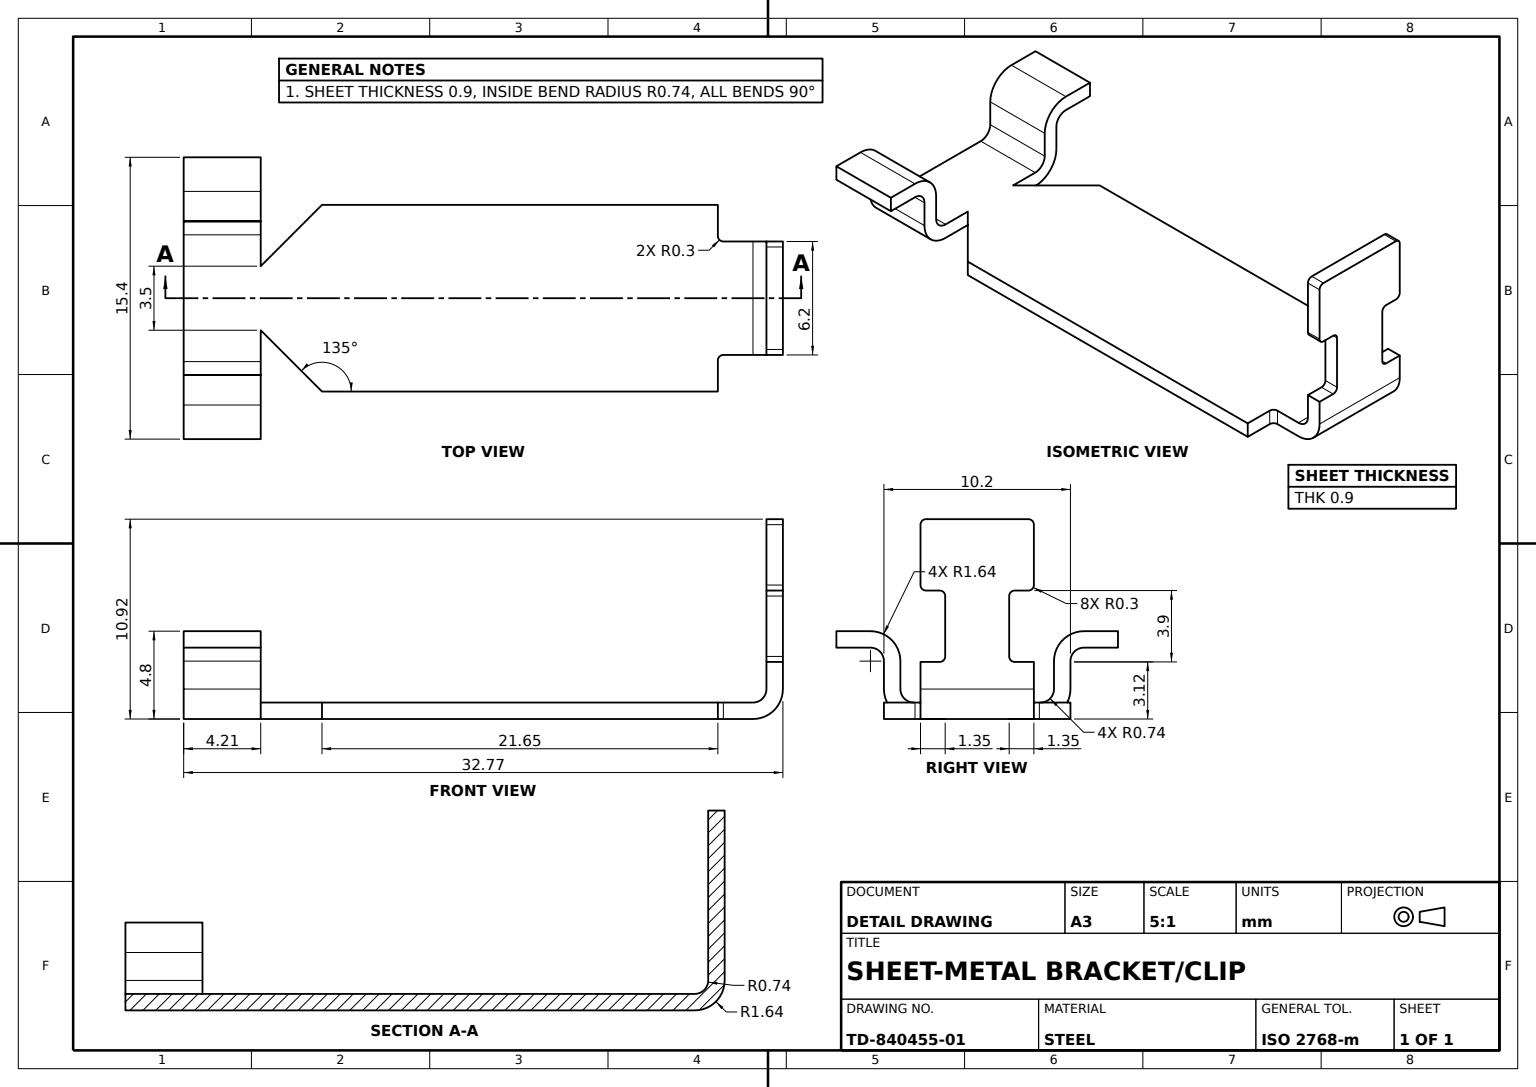
solid
v1 (-2.8,5.46,0)
v2 (-3.1,5.16,0)
e1 v1 v2 CIRCLE(AX(P(-2.8,5.16,0),D(0,0,1),D(0,-1,0)),0.3)
v3 (-2.8,5.46,-0.9)
e2 v3 v1 LINE
v4 (-3.1,5.16,-0.9)
e3 v4 v3 CIRCLE(AX(P(-2.8,5.16,-0.9),D(0,0,-1),D(0,-1,0)),0.3)
e4 v2 v4 LINE
face CYL(AX(P(-2.8,5.16,-0.9),D(0,0,-1),D(0,1,0)),0.3) [-e1 -e2 -e3 -e4]
v5 (-3.1,1.86,-0.9)
e5 v5 v4 LINE
v6 (-3.1,1.86,0)
e6 v5 v6 LINE
e7 v6 v2 LINE
face PLANE(AX(P(-3.1,5.46,-0.9),D(1,0,0),D(0,1,0))) rev [e4 -e5 e6 e7]
v7 (5.8366,-1.56,31.87)
v8 (5.1,-2.2966,31.87)
e8 v7 v8 CIRCLE(AX(P(5.8366,-2.2966,31.87),D(0,0,1),D(0,-1,0)),0.7366)
v9 (5.8366,-0.66,31.87)
e9 v7 v9 LINE
v10 (4.2,-2.2966,31.87)
e10 v9 v10 CIRCLE(AX(P(5.8366,-2.2966,31.87),D(0,0,1),D(0,-1,0)),1.6366)
e11 v8 v10 LINE
face PLANE(AX(P(5.8366,-2.2966,31.87),D(0,0,-1),D(0,1,0))) rev [-e8 e9 e10 -e11]
v11 (2.05,-2.34,0)
v12 (3.1,-2.34,0)
e12 v11 v12 LINE
v13 (1.75,-2.04,0)
e13 v11 v13 CIRCLE(AX(P(2.05,-2.04,0),D(0,0,-1),D(0,-1,0)),0.3)
v14 (1.75,1.26,0)
e14 v14 v13 LINE
v15 (2.05,1.56,0)
e15 v14 v15 CIRCLE(AX(P(2.05,1.26,0),D(0,0,-1),D(0,-1,0)),0.3)
v16 (2.8,1.56,0)
e16 v16 v15 LINE
v17 (3.1,1.86,0)
e17 v16 v17 CIRCLE(AX(P(2.8,1.86,0),D(0,0,1),D(0,-1,0)),0.3)
v18 (3.1,5.16,0)
e18 v18 v17 LINE
v19 (2.8,5.46,0)
e19 v18 v19 CIRCLE(AX(P(2.8,5.16,0),D(0,0,1),D(0,-1,0)),0.3)
e20 v19 v1 LINE
v20 (-2.8,1.56,0)
e21 v6 v20 CIRCLE(AX(P(-2.8,1.86,0),D(0,0,1),D(0,-1,0)),0.3)
v21 (-2.05,1.56,0)
e22 v21 v20 LINE
v22 (-1.75,1.26,0)
e23 v21 v22 CIRCLE(AX(P(-2.05,1.26,0),D(0,0,-1),D(0,-1,0)),0.3)
v23 (-1.75,-2.04,0)
e24 v23 v22 LINE
v24 (-2.05,-2.34,0)
e25 v23 v24 CIRCLE(AX(P(-2.05,-2.04,0),D(0,0,-1),D(0,-1,0)),0.3)
v25 (-3.1,-2.34,0)
e26 v25 v24 LINE
v26 (-3.1,-3.8234,0)
e27 v26 v25 LINE
v27 (3.1,-3.8234,0)
e28 v27 v26 LINE
e29 v12 v27 LINE
face PLANE(AX(P(0,0,0),D(0,0,1),D(1,0,0))) [-e12 e13 -e14 e15 -e16 e17 -e18 e19 e20 e1 -e7 e21 -e22 e23 -e24 e25 -e26 -e27 -e28 -e29]
v28 (-5.8366,-1.56,31.87)
v29 (-5.8366,-1.56,27.6566)
e30 v28 v29 LINE
v30 (-5.1,-2.2966,27.6566)
e31 v29 v30 CIRCLE(AX(P(-5.8366,-2.2966,27.6566),D(0,0,-1),D(0,1,0)),0.7366)
v31 (-5.1,-2.2966,31.87)
e32 v30 v31 LINE
e33 v31 v28 CIRCLE(AX(P(-5.8366,-2.2966,31.87),D(0,0,1),D(0,1,0)),0.7366)
face CYL(AX(P(-5.8366,-2.2966,27.6566),D(0,0,-1),D(0,1,0)),0.7366) rev [e30 e31 e32 e33]
v32 (-5.8366,-0.66,31.87)
v33 (-7.7,-0.66,31.87)
e34 v32 v33 LINE
v34 (-5.8366,-0.66,27.6566)
e35 v34 v32 LINE
v35 (-7.7,-0.66,27.6566)
e36 v35 v34 LINE
e37 v33 v35 LINE
face PLANE(AX(P(0,-0.66,0),D(0,-1,0),D(0,0,-1))) rev [-e34 -e35 -e36 -e37]
v36 (3.4634,-4.56,27.6566)
v37 (3.4634,-5.46,27.6566)
e38 v36 v37 LINE
v38 (1.75,-5.46,27.6566)
e39 v37 v38 LINE
v39 (1.75,-4.56,27.6566)
e40 v39 v38 LINE
e41 v36 v39 LINE
face PLANE(AX(P(5.1,-4.56,27.6566),D(0,0,1),D(0,-1,0))) rev [e38 e39 -e40 -e41]
v40 (-4.2,-3.8234,31.87)
v41 (-3.4634,-4.56,31.87)
e42 v40 v41 CIRCLE(AX(P(-3.4634,-3.8234,31.87),D(0,0,1),D(0,-1,0)),0.7366)
v42 (-5.1,-3.8234,31.87)
e43 v40 v42 LINE
v43 (-3.4634,-5.46,31.87)
e44 v42 v43 CIRCLE(AX(P(-3.4634,-3.8234,31.87),D(0,0,1),D(0,-1,0)),1.6366)
e45 v41 v43 LINE
face PLANE(AX(P(-3.4634,-3.8234,31.87),D(0,0,-1),D(0,1,0))) rev [-e42 e43 e44 -e45]
v44 (1.75,-2.04,-0.9)
v45 (2.05,-2.34,-0.9)
e46 v44 v45 CIRCLE(AX(P(2.05,-2.04,-0.9),D(0,0,1),D(0,-1,0)),0.3)
e47 v13 v44 LINE
e48 v45 v11 LINE
face CYL(AX(P(2.05,-2.04,-0.9),D(0,0,-1),D(0,1,0)),0.3) rev [-e46 -e47 -e13 -e48]
v46 (5.1,-3.8234,31.87)
e49 v46 v8 LINE
v47 (4.2,-3.8234,31.87)
e50 v47 v10 LINE
e51 v47 v46 LINE
face PLANE(AX(P(5.1,-0.66,31.87),D(0,0,1),D(1,0,0))) [e49 e11 -e50 e51]
v48 (-2.05,1.56,-0.9)
v49 (-2.8,1.56,-0.9)
e52 v48 v49 LINE
e53 v49 v5 CIRCLE(AX(P(-2.8,1.86,-0.9),D(0,0,-1),D(0,-1,0)),0.3)
v50 (2.8,5.46,-0.9)
e54 v50 v3 LINE
v51 (3.1,5.16,-0.9)
e55 v50 v51 CIRCLE(AX(P(2.8,5.16,-0.9),D(0,0,-1),D(0,-1,0)),0.3)
v52 (3.1,1.86,-0.9)
e56 v51 v52 LINE
v53 (2.8,1.56,-0.9)
e57 v52 v53 CIRCLE(AX(P(2.8,1.86,-0.9),D(0,0,-1),D(0,-1,0)),0.3)
v54 (2.05,1.56,-0.9)
e58 v53 v54 LINE
v55 (1.75,1.26,-0.9)
e59 v54 v55 CIRCLE(AX(P(2.05,1.26,-0.9),D(0,0,1),D(0,-1,0)),0.3)
e60 v55 v44 LINE
v56 (3.1,-2.34,-0.9)
e61 v45 v56 LINE
v57 (3.1,-3.8234,-0.9)
e62 v56 v57 LINE
v58 (-3.1,-3.8234,-0.9)
e63 v57 v58 LINE
v59 (-3.1,-2.34,-0.9)
e64 v58 v59 LINE
v60 (-2.05,-2.34,-0.9)
e65 v59 v60 LINE
v61 (-1.75,-2.04,-0.9)
e66 v60 v61 CIRCLE(AX(P(-2.05,-2.04,-0.9),D(0,0,1),D(0,-1,0)),0.3)
v62 (-1.75,1.26,-0.9)
e67 v61 v62 LINE
e68 v62 v48 CIRCLE(AX(P(-2.05,1.26,-0.9),D(0,0,1),D(0,-1,0)),0.3)
face PLANE(AX(P(0,0,-0.9),D(0,0,1),D(1,0,0))) rev [e52 e53 e5 e3 -e54 e55 e56 e57 e58 e59 e60 e46 e61 e62 e63 e64 e65 e66 e67 e68]
v63 (-3.4,-4.56,2.6566)
v64 (-3.4,-5.46,2.6566)
e69 v63 v64 LINE
v65 (-5.1,-5.46,2.6566)
e70 v65 v64 LINE
v66 (-5.1,-4.56,2.6566)
e71 v65 v66 LINE
e72 v66 v63 LINE
face PLANE(AX(P(-3.1,-5.46,2.6566),D(0,0,1),D(0,-1,0))) rev [e69 -e70 e71 e72]
v67 (3.4634,-4.56,31.87)
e73 v36 v67 LINE
e74 v67 v47 CIRCLE(AX(P(3.4634,-3.8234,31.87),D(0,0,1),D(0,1,0)),0.7366)
v68 (4.2,-3.8234,27.6566)
e75 v47 v68 LINE
e76 v68 v36 CIRCLE(AX(P(3.4634,-3.8234,27.6566),D(0,0,-1),D(0,1,0)),0.7366)
face CYL(AX(P(3.4634,-3.8234,27.6566),D(0,0,-1),D(1,0,0)),0.7366) rev [e73 e74 e75 e76]
v69 (-3.4634,-5.46,27.6566)
v70 (-5.1,-3.8234,27.6566)
e77 v69 v70 CIRCLE(AX(P(-3.4634,-3.8234,27.6566),D(0,0,-1),D(0,-1,0)),1.6366)
v71 (-4.2,-3.8234,27.6566)
e78 v71 v70 LINE
v72 (-3.4634,-4.56,27.6566)
e79 v72 v71 CIRCLE(AX(P(-3.4634,-3.8234,27.6566),D(0,0,-1),D(0,-1,0)),0.7366)
e80 v72 v69 LINE
face PLANE(AX(P(-3.4634,-3.8234,27.6566),D(0,0,-1),D(0,1,0))) [e77 -e78 -e79 e80]
v73 (-5.1,-4.56,24.3066)
v74 (-1.75,-4.56,27.6566)
e81 v73 v74 LINE
v75 (-5.1,-5.46,24.3066)
e82 v73 v75 LINE
v76 (-1.75,-5.46,27.6566)
e83 v75 v76 LINE
e84 v74 v76 LINE
face PLANE(AX(P(-5.1,-4.56,24.3066),D(0.707106781,0,-0.707106781),D(-0.707106781,0,-0.707106781))) rev [-e81 e82 e83 -e84]
e85 v61 v23 LINE
e86 v24 v60 LINE
face CYL(AX(P(-2.05,-2.04,-0.9),D(0,0,-1),D(0,1,0)),0.3) rev [-e25 -e85 -e66 -e86]
e87 v20 v49 LINE
e88 v48 v21 LINE
face PLANE(AX(P(-3.1,1.56,-0.9),D(0,1,0),D(0,0,1))) rev [e87 -e52 e88 e22]
e89 v70 v42 LINE
e90 v31 v42 LINE
e91 v70 v30 LINE
face PLANE(AX(P(-5.1,0,0),D(-1,0,0),D(0,-1,0))) [e89 -e90 -e32 -e91]
v77 (-4.2,-2.2966,31.87)
e92 v31 v77 LINE
e93 v77 v40 LINE
face PLANE(AX(P(-5.1,-4.56,31.87),D(0,0,1),D(1,0,0))) [-e92 e90 -e43 -e93]
e94 v71 v40 LINE
v78 (-4.2,-2.2966,27.6566)
e95 v71 v78 LINE
e96 v78 v77 LINE
face PLANE(AX(P(-4.2,0,0),D(-1,0,0),D(0,-1,0))) rev [-e94 e95 e96 e93]
v79 (5.1,-5.46,24.3066)
v80 (5.1,-5.46,2.6566)
e97 v79 v80 LINE
e98 v38 v79 LINE
v81 (3.4634,-5.46,31.87)
e99 v37 v81 LINE
e100 v43 v81 LINE
e101 v43 v69 LINE
e102 v76 v69 LINE
e103 v65 v75 LINE
v82 (-3.1,-5.46,2.3566)
e104 v64 v82 CIRCLE(AX(P(-3.4,-5.46,2.3566),D(0,1,0),D(0,0,-1)),0.3)
v83 (-3.1,-5.46,0.7366)
e105 v82 v83 LINE
v84 (3.1,-5.46,0.7366)
e106 v83 v84 LINE
v85 (3.1,-5.46,2.3566)
e107 v84 v85 LINE
v86 (3.4,-5.46,2.6566)
e108 v85 v86 CIRCLE(AX(P(3.4,-5.46,2.3566),D(0,1,0),D(0,0,-1)),0.3)
e109 v86 v80 LINE
face PLANE(AX(P(0,-5.46,0),D(0,-1,0),D(0,0,-1))) [-e97 -e98 -e39 e99 -e100 e101 -e102 -e83 -e103 e70 e104 e105 e106 e107 e108 e109]
v87 (5.1,-2.2966,27.6566)
v88 (5.8366,-1.56,27.6566)
e110 v87 v88 CIRCLE(AX(P(5.8366,-2.2966,27.6566),D(0,0,-1),D(0,-1,0)),0.7366)
e111 v88 v7 LINE
e112 v8 v87 LINE
face CYL(AX(P(5.8366,-2.2966,31.87),D(0,0,1),D(0,1,0)),0.7366) rev [e110 e111 e8 e112]
v89 (3.1,-4.56,2.3566)
e113 v89 v85 LINE
v90 (3.4,-4.56,2.6566)
e114 v90 v89 CIRCLE(AX(P(3.4,-4.56,2.3566),D(0,-1,0),D(0,0,-1)),0.3)
e115 v86 v90 LINE
face CYL(AX(P(3.4,-5.46,2.3566),D(0,-1,0),D(0,0,-1)),0.3) rev [-e108 -e113 -e114 -e115]
v91 (7.7,-1.56,27.6566)
e116 v88 v91 LINE
v92 (7.7,-1.56,31.87)
e117 v91 v92 LINE
e118 v92 v7 LINE
face PLANE(AX(P(0,-1.56,0),D(0,1,0),D(0,0,1))) rev [e116 e117 e118 -e111]
v93 (-7.7,-1.56,27.6566)
e119 v35 v93 LINE
v94 (-7.7,-1.56,31.87)
e120 v94 v93 LINE
e121 v33 v94 LINE
face PLANE(AX(P(-7.7,-0.66,31.87),D(-1,0,0),D(0,-1,0))) [e119 -e120 -e121 e37]
face CYL(AX(P(-3.4634,-3.8234,31.87),D(0,0,1),D(-1,0,0)),1.6366) [-e89 -e77 -e101 -e44]
v95 (5.1,-4.56,2.6566)
e122 v90 v95 LINE
e123 v80 v95 LINE
face PLANE(AX(P(3.1,-5.46,2.6566),D(0,0,1),D(0,-1,0))) rev [e115 e122 -e123 -e109]
e124 v81 v46 CIRCLE(AX(P(3.4634,-3.8234,31.87),D(0,0,1),D(0,1,0)),1.6366)
v96 (5.1,-3.8234,27.6566)
e125 v96 v37 CIRCLE(AX(P(3.4634,-3.8234,27.6566),D(0,0,-1),D(0,1,0)),1.6366)
e126 v46 v96 LINE
face CYL(AX(P(3.4634,-3.8234,27.6566),D(0,0,-1),D(1,0,0)),1.6366) [-e124 -e99 -e125 -e126]
e127 v22 v62 LINE
face PLANE(AX(P(-1.75,1.56,-0.9),D(1,0,0),D(0,1,0))) rev [e85 e24 e127 -e67]
e128 v68 v96 LINE
face PLANE(AX(P(3.4634,-3.8234,27.6566),D(0,0,1),D(0,-1,0))) rev [-e38 -e76 e128 e125]
e129 v56 v12 LINE
face PLANE(AX(P(1.75,-2.34,-0.9),D(0,-1,0),D(0,0,-1))) rev [e48 e12 -e129 -e61]
v97 (5.1,-4.56,24.3066)
e130 v97 v95 LINE
e131 v97 v79 LINE
face PLANE(AX(P(5.1,-5.46,0),D(1,0,0),D(0,0,-1))) [e123 -e130 e131 e97]
v98 (7.7,-0.66,31.87)
e132 v98 v9 LINE
e133 v98 v92 LINE
face PLANE(AX(P(5.1,-0.66,31.87),D(0,0,1),D(0,-1,0))) [e132 -e9 -e118 -e133]
e134 v74 v72 LINE
face PLANE(AX(P(-1.75,-4.56,27.6566),D(0,0,1),D(0,-1,0))) rev [e84 e102 -e80 -e134]
v99 (3.1,-4.56,0.7366)
e135 v27 v99 CIRCLE(AX(P(3.1,-3.8234,0.7366),D(-1,0,0),D(0,0,-1)),0.7366)
e136 v99 v84 LINE
e137 v57 v84 CIRCLE(AX(P(3.1,-3.8234,0.7366),D(-1,0,0),D(0,0,1)),1.6366)
e138 v57 v27 LINE
face PLANE(AX(P(3.1,-3.8234,0.7366),D(1,0,0),D(0,0,-1))) [e135 e136 -e137 e138]
e139 v83 v58 CIRCLE(AX(P(-3.1,-3.8234,0.7366),D(1,0,0),D(0,0,-1)),1.6366)
v100 (-3.1,-4.56,0.7366)
e140 v83 v100 LINE
e141 v100 v26 CIRCLE(AX(P(-3.1,-3.8234,0.7366),D(1,0,0),D(0,0,-1)),0.7366)
e142 v26 v58 LINE
face PLANE(AX(P(-3.1,-3.8234,0.7366),D(-1,0,0),D(0,0,1))) [-e139 e140 e141 e142]
e143 v66 v73 LINE
face PLANE(AX(P(-5.1,-5.46,31.87),D(-1,0,0),D(0,0,1))) [-e143 -e71 e103 -e82]
e144 v99 v89 LINE
e145 v100 v99 LINE
v101 (-3.1,-4.56,2.3566)
e146 v101 v100 LINE
e147 v101 v63 CIRCLE(AX(P(-3.4,-4.56,2.3566),D(0,-1,0),D(0,0,-1)),0.3)
e148 v41 v72 LINE
e149 v41 v67 LINE
e150 v39 v97 LINE
face PLANE(AX(P(0,-4.56,0),D(0,-1,0),D(0,0,-1))) rev [e114 -e144 -e145 -e146 e147 -e72 e143 e81 e134 -e148 e149 -e73 e41 e150 e130 -e122]
e151 v17 v52 LINE
e152 v53 v16 LINE
face CYL(AX(P(2.8,1.86,-0.9),D(0,0,1),D(0,-1,0)),0.3) [-e151 -e17 -e152 -e57]
e153 v19 v50 LINE
face PLANE(AX(P(-5.1,5.46,-0.9),D(0,1,0),D(0,0,1))) [e2 -e20 e153 e54]
v102 (4.2,-2.2966,27.6566)
e154 v10 v102 LINE
v103 (5.8366,-0.66,27.6566)
e155 v103 v9 LINE
e156 v102 v103 CIRCLE(AX(P(5.8366,-2.2966,27.6566),D(0,0,-1),D(0,-1,0)),1.6366)
face CYL(AX(P(5.8366,-2.2966,31.87),D(0,0,1),D(0,1,0)),1.6366) [-e154 -e10 -e155 -e156]
e157 v88 v103 LINE
v104 (7.7,-0.66,27.6566)
e158 v103 v104 LINE
e159 v104 v91 LINE
face PLANE(AX(P(7.7,-0.66,27.6566),D(0,0,-1),D(0,1,0))) [e157 e158 e159 -e116]
e160 v104 v98 LINE
face PLANE(AX(P(7.7,-0.66,31.87),D(1,0,0),D(0,1,0))) [-e117 -e159 e160 e133]
e161 v51 v18 LINE
face PLANE(AX(P(3.1,5.46,-0.9),D(-1,0,0),D(0,-1,0))) rev [-e56 e161 e18 e151]
e162 v102 v68 LINE
face PLANE(AX(P(4.2,0,0),D(1,0,0),D(0,1,0))) rev [e154 e162 -e75 e50]
e163 v15 v54 LINE
e164 v55 v14 LINE
face CYL(AX(P(2.05,1.26,-0.9),D(0,0,-1),D(0,1,0)),0.3) rev [-e163 -e15 -e164 -e59]
e165 v77 v32 CIRCLE(AX(P(-5.8366,-2.2966,31.87),D(0,0,1),D(0,1,0)),1.6366)
e166 v34 v78 CIRCLE(AX(P(-5.8366,-2.2966,27.6566),D(0,0,-1),D(0,1,0)),1.6366)
face CYL(AX(P(-5.8366,-2.2966,27.6566),D(0,0,-1),D(0,1,0)),1.6366) [-e165 -e96 -e166 e35]
e167 v28 v32 LINE
face PLANE(AX(P(-5.8366,-2.2966,31.87),D(0,0,1),D(0,-1,0))) [-e33 e92 e165 -e167]
e168 v59 v25 LINE
face PLANE(AX(P(-1.75,-2.34,-0.9),D(0,-1,0),D(0,0,-1))) rev [e168 e26 e86 -e65]
face PLANE(AX(P(3.1,-2.34,-0.9),D(-1,0,0),D(0,-1,0))) rev [e29 -e138 -e62 e129]
face CYL(AX(P(-2.8,1.86,-0.9),D(0,0,1),D(0,-1,0)),0.3) [-e53 -e87 -e21 -e6]
face PLANE(AX(P(1.75,-4.56,27.6566),D(-0.707106781,0,-0.707106781),D(-0.707106781,0,0.707106781))) rev [-e131 -e150 e40 e98]
e169 v30 v78 LINE
e170 v29 v34 LINE
face PLANE(AX(P(-5.8366,-2.2966,27.6566),D(0,0,1),D(0,-1,0))) rev [e166 -e169 -e31 e170]
face PLANE(AX(P(3.1,1.56,-0.9),D(0,1,0),D(0,0,1))) rev [-e58 e152 e16 e163]
face CYL(AX(P(-6.536371,-3.8234,0.7366),D(1,0,0),D(0,0,-1)),0.7366) rev [-e135 e28 -e141 e145]
face CYL(AX(P(-2.05,1.26,-0.9),D(0,0,-1),D(0,1,0)),0.3) rev [-e127 -e23 -e88 -e68]
e171 v87 v96 LINE
face PLANE(AX(P(5.1,0,0),D(1,0,0),D(0,1,0))) [e126 -e171 -e112 -e49]
e172 v82 v101 LINE
face CYL(AX(P(-3.4,-5.46,2.3566),D(0,-1,0),D(0,0,-1)),0.3) rev [-e147 -e172 -e104 -e69]
face CYL(AX(P(2.8,5.16,-0.9),D(0,0,-1),D(0,1,0)),0.3) [-e19 -e161 -e55 -e153]
face PLANE(AX(P(3.1,-5.46,-2.610707),D(-1,0,0),D(0,0,1))) rev [e144 e113 -e107 -e136]
e173 v67 v81 LINE
face PLANE(AX(P(5.1,-5.46,31.87),D(0,0,1),D(0,-1,0))) [e100 -e173 -e149 e45]
e174 v87 v102 LINE
face PLANE(AX(P(5.1,-4.56,27.6566),D(0,0,-1),D(0,1,0))) [-e174 e171 -e128 -e162]
face CYL(AX(P(-3.4634,-3.8234,31.87),D(0,0,1),D(-1,0,0)),0.7366) rev [e148 e79 e94 e42]
face CYL(AX(P(-6.536371,-3.8234,0.7366),D(1,0,0),D(0,0,-1)),1.6366) [-e63 e137 -e106 e139]
e175 v93 v29 LINE
face PLANE(AX(P(-7.7,-0.66,27.6566),D(0,0,-1),D(0,1,0))) [-e119 e36 -e170 -e175]
e176 v28 v94 LINE
face PLANE(AX(P(-5.1,-0.66,31.87),D(0,0,1),D(0,-1,0))) [e121 -e176 e167 e34]
face PLANE(AX(P(1.75,1.56,-0.9),D(-1,0,0),D(0,-1,0))) rev [e47 -e60 e164 e14]
face PLANE(AX(P(3.4634,-3.8234,31.87),D(0,0,1),D(0,-1,0))) [-e74 e173 e124 -e51]
face PLANE(AX(P(0,-0.66,0),D(0,1,0),D(0,0,1))) [-e132 -e160 -e158 e155]
face PLANE(AX(P(5.8366,-2.2966,27.6566),D(0,0,-1),D(0,1,0))) [e156 -e157 -e110 e174]
face PLANE(AX(P(-5.1,-0.66,27.6566),D(0,0,-1),D(0,1,0))) [-e95 e78 e91 e169]
face PLANE(AX(P(-3.1,-2.34,-0.9),D(1,0,0),D(0,1,0))) rev [-e142 e27 -e168 -e64]
face PLANE(AX(P(0,-1.56,0),D(0,-1,0),D(0,0,-1))) [-e30 e176 e120 e175]
face PLANE(AX(P(-3.1,-5.46,-2.610707),D(1,0,0),D(0,0,-1))) rev [e146 -e140 -e105 e172]
